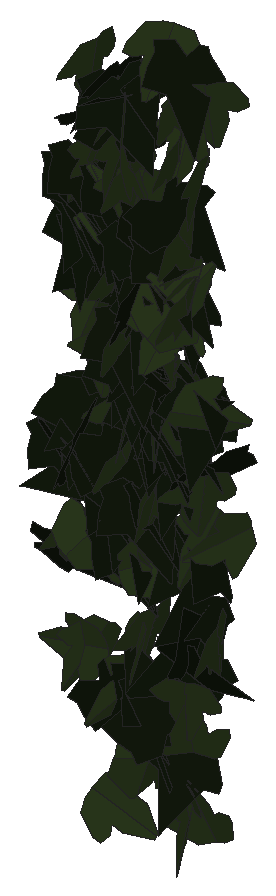
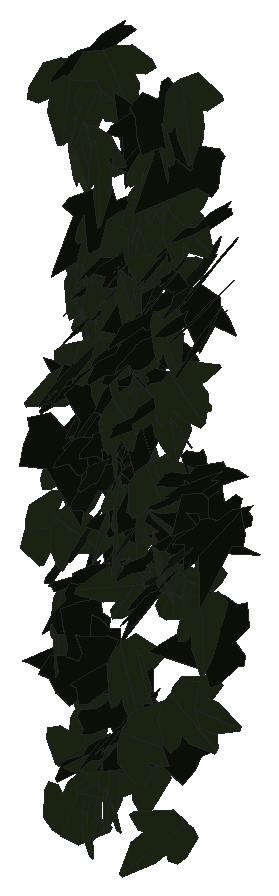
# SketchUp Ruby script. Lengths in inches.
U = 1.inch
M = Sketchup.active_model
def pt(a) = Geom::Point3d.new(a.map { |v| v * U })
def face(e, loops, mat)
  f = e.add_face(loops[0].map { |a| pt(a) })
  loops[1..].each { |l| e.add_face(l.map { |a| pt(a) }).erase! }
  f.material = f.back_material = mat if mat
  f
end
# faces: each face lists its corners as indices into pts; further lists are holes
def faces(e, pts, list, mat = nil) = list.each { |f| face(e, (f[0].is_a?(Array) ? f : [f]).map { |l| l.map { |i| pts[i] } }, mat) }
# xy, xz, yz: faces in a plane at the given z, y or x. An outline is a flat list of corners, or four numbers for a rectangle; further outlines are holes
def ring(l) = l.size == 4 ? [[l[0], l[1]], [l[2], l[1]], [l[2], l[3]], [l[0], l[3]]] : l.each_slice(2).to_a
def flat(e, list, mat, &to3) = list.each { |f| face(e, (f[0].is_a?(Array) ? f : [f]).map { |l| ring(l).map { |u, v| to3.(u, v) } }, mat) }
def xy(e, z, list, mat = nil) = flat(e, list, mat) { |x, y| [x, y, z] }
def xz(e, y, list, mat = nil) = flat(e, list, mat) { |x, z| [x, y, z] }
def yz(e, x, list, mat = nil) = flat(e, list, mat) { |y, z| [x, y, z] }
def lines(e, pts, list) = list.each { |a, b| e.add_line(pt(pts[a]), pt(pts[b])) }
# prism: a flat outline (further loops are holes) pulled along v
def prism(e, loops, v, mat = nil)
  f = face(e, loops, mat); d = Geom::Vector3d.new(v.map { |x| x * U })
  f.pushpull(f.normal.samedirection?(d) ? d.length : -d.length)
end
def box(e, o, s, mat = nil) = prism(e, [[o, [o[0] + s[0], o[1], o[2]], [o[0] + s[0], o[1] + s[1], o[2]], [o[0], o[1] + s[1], o[2]]]], [0, 0, s[2]], mat)
def at(x, y, z, deg = 0) = Geom::Transformation.translation(pt([x, y, z])) * Geom::Transformation.rotation(ORIGIN, Z_AXIS, deg.degrees)
def axes(o, x, y, z) = Geom::Transformation.new([*x, 0, *y, 0, *z, 0, *pt(o).to_a, 1])
def part(name) = M.definitions.add(name)
# library, detail: a bought-in or finely detailed component or shape, given as its bounding box
def library(name, o, s) = part(name).tap { |d| box(d.entities, o, s) }
def detail(e, o, s) = box(e.add_group.entities, o, s)
def put(e, d, t, mat = nil) = e.add_instance(d, t).tap { |i| i.material = mat if mat }
def group(e, t, mat = nil) = e.add_group.tap { |g| g.transformation = t; g.material = mat if mat }.entities
root = M.entities
M.materials.add("efeu1").color = [18, 25, 13]
M.materials.add("efeu2").color = [43, 57, 29]
c1 = part("ivyleaf_10")
p = [[0,0.5,-0.03],[-0.0625,2.02,-0.43],[-0.19,2.01,-0.46],[-0.54,1.05,-0.29],[-0.52,0.625,-0.18],[-0.83,0.76,-0.28],
  [-1.16,0.64,-0.33],[-1.15,0.33,-0.24],[-0.77,-0.39,0.02],[-0.3,-0.51,0.16],[0.04,-0.48,0.23],[-0.02,2.01,-0.4375],
  [-0.06,2.01,-0.43],[0.04,-0.49,0.23],[0.67,-0.49,0.14],[1.38,0.36,-0.2],[1.375,0.51,-0.24],[0.81,0.65,-0.19],
  [0.62,0.59,-0.15],[0.6,1.09,-0.28],[0.5,1.23,-0.31]]
faces(c1.entities,p,[[0,1,2,3,4,5,6,7,8,9,10],[11,12,0,13,14,15,16,17,18,19,20]],"efeu2")
c2 = part("ivyleaf_9")
p = [[1.54,2.16,1.25],[1.36,2.04,1.19],[-0.21,0.99,0.68],[-0.71,1.11,0.82],[-0.85,0.86,0.67],[-0.8,0.17,0.21],
  [-0.9,-0.01,0.1],[-0.67,-0.16,-0.02],[-0.08,-0.08,-0.05],[-0.03,-0.6,-0.4],[0.65,-0.88,-0.66],[0.83,-0.6,-0.49],
  [1.29,-0.42,-0.43],[1.8125,-0.07,-0.26],[1.21,0.44,0.15]]
faces(c2.entities,p,[[0,1,2,3,4,5,6,7,8,9,10,11,12,13,14]],"efeu1")
put(root,c1,axes([526.44,133.65,198.45],[0.31134,0.45715,-0.77984],[0.46763,0.62441,0.55273],[0.7736,-0.56142,-0.02027]))
put(root,c2,axes([527.04,134.69,195.85],[-0.12477,-0.77393,0.1001],[0.00797,-0.10263,-0.78355],[0.78033,-0.12269,0.02401]))
put(root,c1,axes([525.07,133.81,197.625],[-0.04112,-0.53898,-0.66297],[0.07443,0.65896,-0.54033],[0.85117,-0.08366,0.01522]))
put(root,c2,axes([526.71,134.58,188.76],[0.15218,0.40988,0.69617],[-0.23852,-0.65404,0.43722],[0.77186,-0.28292,-0.00215]))
put(root,c2,axes([525.39,133.55,198.23],[0.12896,0.35513,0.7991],[0.23978,0.76242,-0.37752],[-0.84094,0.27185,0.0149]))
put(root,c2,axes([525.3,134.86,194.29],[0.07511,-0.51258,0.6061],[0.11333,-0.59564,-0.51778],[0.78565,0.13493,0.01675]))
put(root,c1,axes([526.84,134.16,198.89],[0.0292,-0.79802,-0.29345],[0.04088,0.2946,-0.79708],[0.84928,0.01325,0.04846]))
put(root,c2,axes([526.11,134.29,186.49],[-0.63905,-0.58234,0.19141],[0.15334,0.11584,0.86442],[-0.5935,0.65697,0.01725]))
put(root,c2,axes([525.05,134.49,197.51],[-0.30421,-0.72268,-0.38636],[0.14579,0.35783,-0.78409],[0.8064,-0.33732,-0.004]))
put(root,c1,axes([526.21,134.41,198.08],[0.69804,0.27879,-0.29682],[-0.28882,-0.07628,-0.7509],[-0.28706,0.75468,0.03375]))
put(root,c2,axes([524.98,134.49,196.68],[-0.49657,-0.45951,-0.41466],[0.2841,0.30309,-0.67609],[0.54989,-0.57154,-0.02515]))
put(root,c2,axes([522.87,134.07,193.61],[0.6998,0.05372,-0.52183],[-0.5196,-0.04871,-0.70182],[-0.07217,0.87158,-0.00706]))
put(root,c2,axes([526.52,134.65,205.43],[0.02662,-0.84739,-0.0878],[-0.00156,0.0878,-0.84781],[0.85192,0.02664,0.00119]))
put(root,c2,axes([525.16,134.75,200.14],[0.2318,-0.75724,0.24907],[0.10266,-0.22887,-0.79136],[0.79051,0.25177,0.02974]))
put(root,c2,axes([525.83,134.49,199.98],[0.22908,-0.75036,-0.18724],[0.01233,0.1988,-0.7816],[0.77327,0.21913,0.06793]))
put(root,c2,axes([526.51,134.86,185.75],[-0.29078,-0.72484,0.15526],[-0.03642,-0.1526,-0.78067],[0.74039,-0.29218,0.02257]))
put(root,c1,axes([526.43,134.83,184.1],[0.2052,-0.48673,0.64315],[0.43004,-0.49542,-0.51213],[0.68236,0.45859,0.12936]))
put(root,c1,axes([523.77,134.41,204.93],[-0.06427,-0.83592,-0.05428],[0.00649,0.05394,-0.83838],[0.83766,-0.06455,0.00233]))
put(root,c2,axes([523.67,133.7,193.88],[-0.2778,0.34432,-0.75773],[-0.56075,0.51287,0.43864],[0.61504,0.62313,0.05767]))
put(root,c2,axes([523.3,134.75,194.66],[-0.39034,-0.6629,-0.13299],[0.11802,0.08441,-0.7671],[0.66573,-0.40365,0.05801]))
put(root,c1,axes([527.02,134.6,202.5625],[0.32017,-0.74024,0.1502],[0.09499,-0.12238,-0.80562],[0.74932,0.3318,0.03795]))
put(root,c1,axes([523.74,134.38,187.97],[0.13,0.01854,-0.7798],[-0.76876,0.13692,-0.1249],[0.13209,0.77862,0.04053]))
put(root,c2,axes([526.375,134.47,195.54],[0.56041,-0.56093,-0.02549],[-0.01663,0.01942,-0.7929],[0.56126,0.56065,0.00196]))
put(root,c1,axes([525.16,134.4,188.66],[0.50138,-0.62547,-0.22873],[-0.14537,0.17662,-0.80161],[0.64992,0.52202,-0.00284]))
put(root,c1,axes([524.48,134.71,202.5],[0.15512,-0.7754,0.28206],[0.09573,-0.26815,-0.78981],[0.81954,0.17809,0.03887]))
put(root,c1,axes([527.09,133.92,196.01],[-0.23757,-0.29741,-0.81773],[0.54563,0.60938,-0.38016],[0.67781,-0.59479,0.01941]))
put(root,c1,axes([526.73,134.38,187.72],[-0.7022,-0.23546,0.06145],[-0.0567,-0.0242,-0.74061],[0.23665,-0.70447,0.00491]))
put(root,c1,axes([523.58,134.82,188.09],[-0.15948,-0.64811,0.46925],[-0.07214,-0.46488,-0.66659],[0.79689,-0.17179,0.03357]))
put(root,c1,axes([523.62,133.95,191.07],[0.3816,0.27253,-0.68362],[0.46599,0.50654,0.46206],[0.56961,-0.59697,0.07998]))
put(root,c2,axes([524.44,134.53,204.55],[-0.33256,0.6112,-0.43787],[0.12378,-0.42775,-0.69109],[-0.7416,-0.34548,0.081]))
put(root,c1,axes([524.07,134.5,191.02],[-0.01847,-0.04676,0.81979],[0.82026,0.03653,0.02056],[-0.03764,0.81918,0.04588]))
put(root,c1,axes([524.74,134.63,195.1],[0.48288,-0.61856,0.09808],[0.05435,-0.08199,-0.78469],[0.62392,0.48588,-0.00755]))
put(root,c1,axes([527.17,134.5,193.68],[-0.42602,-0.67903,0.04435],[-0.02532,-0.03647,-0.8016],[0.68,-0.42676,-0.00206]))
put(root,c2,axes([523.24,134.63,201.55],[0.15948,-0.78413,-0.19331],[0.01342,0.19959,-0.79853],[0.8075,0.15155,0.05145]))
put(root,c1,axes([524.23,134.67,198.63],[0.18506,-0.79542,0.11417],[0.03765,-0.10845,-0.81658],[0.80269,0.18848,0.01198]))
put(root,c2,axes([526.82,135.16,190.1],[0.19036,-0.31801,-0.71542],[0.32402,-0.63825,0.36992],[-0.71272,-0.3751,-0.02291]))
put(root,c1,axes([526.44,134.45,199.09],[-0.27492,-0.77628,-0.1375],[0.05103,0.12779,-0.82351],[0.78671,-0.27956,0.00536]))
put(root,c2,axes([524.61,134.27,202.73],[-0.45695,-0.09896,0.70036],[0.70193,0.03932,0.46352],[-0.08718,0.83532,0.06115]))
put(root,c2,axes([525.76,134.51,195.24],[0.1186,-0.16988,0.8106],[0.77965,-0.25337,-0.16717],[0.27942,0.77907,0.12239]))
put(root,c2,axes([525.26,134.64,187.14],[0.30181,-0.71253,-0.15559],[-0.03025,0.15602,-0.77314],[0.72869,0.30159,0.03235]))
put(root,c1,axes([524.39,134.1,184.01],[0.27208,0.45753,0.6261],[0.30847,0.5449,-0.53225],[-0.71146,0.41123,0.00867]))
put(root,c1,axes([523.51,134.97,201.84],[0.05713,-0.63947,0.49199],[0.05244,-0.48924,-0.64198],[0.80512,0.07724,0.0069]))
put(root,c2,axes([524.5,134.5,204.14],[-0.13046,-0.62877,-0.56176],[0.07364,0.55778,-0.64141],[0.83994,-0.14656,-0.03102]))
put(root,c2,axes([525.72,134.99,194.38],[0.21799,-0.64149,0.45015],[0.21823,-0.39907,-0.67437],[0.75267,0.30149,0.06516]))
put(root,c2,axes([525.13,134.57,192.73],[-0.20018,-0.57923,-0.54341],[0.22082,0.49772,-0.61187],[0.76292,-0.29604,0.03452]))
put(root,c2,axes([523.91,135.04,199.85],[0.1509,-0.68165,0.39536],[0.11026,-0.38032,-0.6978],[0.78025,0.18558,0.02215]))
put(root,c2,axes([524.2,134.27,194.06],[-0.00202,-0.34703,-0.79748],[0.20834,0.77407,-0.33738],[0.84439,-0.19182,0.08133]))
put(root,c1,axes([525.22,134.06,185.55],[-0.15506,-0.17635,-0.85934],[0.63317,0.5815,-0.23358],[0.60717,-0.65144,0.02413]))
put(root,c2,axes([526.9,135.07,196.23],[0.08953,-0.6586,0.46324],[0.21512,-0.42959,-0.65233],[0.77594,0.19509,0.12741]))
put(root,c2,axes([525.14,134.33,196.5],[-0.46457,0.53391,0.36751],[-0.28183,0.24078,-0.70607],[-0.58368,-0.54121,0.04842]))
put(root,c1,axes([525.34,135.0625,194.79],[0.09278,-0.30387,0.75573],[0.55167,-0.53617,-0.28332],[0.59928,0.54062,0.1438]))
put(root,c2,axes([524.05,134.9,192.87],[-0.63778,-0.06359,0.51912],[-0.5109,-0.09932,-0.63985],[0.11184,-0.81633,0.03741]))
put(root,c2,axes([526.8,135.22,191.27],[-0.06868,-0.54907,0.63036],[0.13004,-0.63181,-0.53616],[0.82579,0.05383,0.13685]))
put(root,c2,axes([523.04,135.04,200.21],[0.21505,-0.71302,0.35637],[0.1455,-0.3278,-0.74365],[0.78372,0.2565,0.04027]))
put(root,c1,axes([526.86,135.15,192.16],[-0.08458,-0.55649,0.62678],[0.18393,-0.62693,-0.53181],[0.81774,0.08345,0.18444]))
put(root,c1,axes([526.36,134.49,196.79],[-0.76986,0.10412,0.33772],[-0.33872,0.01357,-0.77632],[-0.10083,-0.84057,0.0293]))
put(root,c2,axes([526.78,134.99,188.44],[-0.00772,-0.02878,-0.80378],[-0.33633,-0.73005,0.02937],[-0.7306,0.33638,-0.00502]))
put(root,c1,axes([526.625,134.81,199],[-0.00456,-0.80127,0.13001],[-0.01809,-0.12988,-0.8011],[0.81155,-0.0074,-0.01712]))
put(root,c2,axes([525.87,134.67,199.47],[0.33139,-0.69883,-0.2613],[0.03236,0.29911,-0.75891],[0.74538,0.29771,0.14911]))
put(root,c1,axes([526.59,134.86,185.74],[-0.4981,-0.6166,-0.17507],[-0.10956,-0.13655,0.79266],[-0.63154,0.51001,0.00057]))
put(root,c2,axes([522.23,134.52,190.29],[0.66453,-0.16089,0.42007],[0.41368,-0.07577,-0.68343],[0.17669,0.78251,0.02019]))
put(root,c1,axes([525.2,134.93,199.42],[0.2443,-0.70608,0.29635],[0.18362,-0.24797,-0.74219],[0.74341,0.29328,0.08593]))
put(root,c2,axes([524.3,134.59,191.37],[0.34255,-0.65099,-0.38619],[-0.14454,0.35984,-0.73478],[0.743,0.37013,0.03511]))
put(root,c1,axes([524.59,135.24,187.03],[-0.07132,-0.4363,0.75754],[-0.11677,-0.74849,-0.44209],[0.86637,-0.1368,0.00278]))
put(root,c2,axes([523.2,134.84,199.88],[-0.61832,-0.20887,-0.52588],[0.48542,0.20449,-0.65196],[0.29077,-0.78553,-0.02989]))
put(root,c2,axes([523.73,134.03,203.33],[0.5432,0.54528,0.27712],[0.04991,0.32988,-0.74691],[-0.60962,0.51287,0.18578]))
put(root,c1,axes([524.14,134.72,196.48],[-0.64908,-0.41453,0.17804],[-0.12739,-0.13085,-0.76908],[0.43279,-0.66021,0.04064]))
put(root,c2,axes([526.19,134.93,194.29],[-0.66044,-0.28531,-0.38832],[0.36993,0.12198,-0.71878],[0.30879,-0.75637,0.03056]))
put(root,c2,axes([526.2,134.59,188.3],[0.5605,-0.13073,0.50882],[0.48668,-0.15095,-0.5749],[0.19782,0.74181,-0.02732]))
put(root,c2,axes([524.72,135.17,191.28],[0.11723,-0.67059,0.38038],[0.04206,-0.37861,-0.68045],[0.76981,0.12281,-0.02075]))
put(root,c1,axes([524.23,134.8,192.39],[0.30376,-0.70834,0.0458],[0.02472,-0.03923,-0.77069],[0.70939,0.30468,0.00725]))
put(root,c2,axes([525.01,134.38,196.31],[0.50677,0.45524,-0.40751],[-0.38605,-0.17179,-0.672],[-0.47358,0.62719,0.11172]))
put(root,c2,axes([523.56,135.28,192.25],[-0.15692,-0.61523,0.48098],[0.12926,-0.50429,-0.60287],[0.77016,-0.04072,0.19919]))
put(root,c2,axes([525.33,134.99,195.2],[-0.27321,-0.74959,-0.16478],[0.04275,0.15977,-0.79769],[0.76629,-0.27616,-0.01424]))
put(root,c2,axes([522.51,134.74,193.6],[0.08383,-0.67692,-0.36171],[0.05206,0.36804,-0.6767],[0.76573,0.04909,0.0856]))
put(root,c2,axes([524.97,134.57,200.1],[0.12897,-0.58757,-0.57627],[0.01112,0.5845,-0.59347],[0.82292,0.08419,0.09833]))
put(root,c1,axes([527.08,134.84,183.72],[-0.7173,-0.11572,-0.25862],[-0.25255,-0.05795,0.7264],[-0.12843,0.76029,0.016]))
put(root,c2,axes([524.08,134.36,187.08],[-0.00997,-0.00816,-0.79816],[0.36214,0.7113,-0.01179],[0.71133,-0.36224,-0.00518]))
put(root,c2,axes([526.18,134.95,194.74],[-0.07352,-0.74961,-0.20474],[-0.00945,0.2065,-0.75267],[0.77701,-0.06842,-0.02853]))
put(root,c2,axes([525.37,135.11,186.9],[0.12094,-0.86457,0.05842],[0.01008,-0.05758,-0.87298],[0.86648,0.12135,0.002]))
put(root,c1,axes([524.89,134.41,202.24],[-0.27544,0.69997,0.30219],[-0.14771,0.26623,-0.7513],[-0.74797,-0.31034,0.03709]))
put(root,c1,axes([525.61,134.47,192.89],[0.17255,-0.71204,-0.44932],[0.00788,0.46,-0.72594],[0.84191,0.14163,0.09888]))
put(root,c1,axes([526.62,134.84,199.35],[0.53244,-0.61331,-0.0153],[-0.01234,0.00955,-0.81218],[0.61337,0.53258,-0.00306]))
put(root,c2,axes([524.33,135.2,192.25],[-0.15891,-0.73599,0.14313],[0.01693,-0.14979,-0.75147],[0.74959,-0.15265,0.04732]))
put(root,c1,axes([524.25,134.74,200.02],[0.36318,0.69126,0.2309],[-0.16386,-0.17393,0.77843],[0.71014,-0.39365,0.06152]))
put(root,c1,axes([524.625,134.53,193.6],[-0.16599,-0.69127,-0.35294],[0.07547,0.34484,-0.71089],[0.77248,-0.18223,-0.00639]))
put(root,c2,axes([523.79,134.96,200.9],[0.30086,-0.772,-0.06699],[-0.01959,0.06427,-0.82854],[0.77465,0.30146,0.00507]))
put(root,c2,axes([527.42,134.55,194.34],[0.04036,0.75873,-0.26869],[-0.04809,-0.26628,-0.75913],[-0.80346,0.05405,0.03194]))
put(root,c2,axes([522.51,135,200.77],[0.30613,-0.76598,-0.00762],[-0.00116,0.00774,-0.82489],[0.76602,0.30613,0.0018]))
put(root,c2,axes([522.82,135.4,198.45],[-0.11527,-0.45927,0.64404],[-0.07346,-0.64181,-0.47083],[0.7876,-0.12708,0.05035]))
put(root,c1,axes([524.41,134.6,203.65],[0.57685,-0.50635,-0.3483],[-0.14174,0.3552,-0.75113],[0.598,0.57262,0.15794]))
put(root,c1,axes([525.82,134.58,185.68],[0.08938,-0.76116,-0.33495],[0.04447,0.34077,-0.76252],[0.83041,0.06368,0.07688]))
put(root,c1,axes([526.48,134.47,200.47],[-0.00699,-0.65575,-0.47411],[0.07301,0.47168,-0.65347],[0.80588,-0.04842,0.05509]))
put(root,c1,axes([527.42,134.65,189.46],[0.17474,-0.73806,-0.29627],[0.02007,0.30734,-0.75378],[0.79505,0.15446,0.08414]))
put(root,c2,axes([523.38,135.42,194.3125],[-0.46747,-0.46715,0.42333],[-0.11137,-0.45753,-0.62787],[0.62051,-0.43405,0.20623]))
put(root,c2,axes([525.75,135.32,193.72],[0.03386,-0.50671,0.63045],[0.29979,-0.5782,-0.48081],[0.75123,0.25358,0.16346]))
put(root,c2,axes([525.05,134.9,192.48],[0.44622,-0.62635,-0.09543],[-0.04331,0.08629,-0.7689],[0.63209,0.44808,0.01468]))
put(root,c2,axes([525.93,134.49,201.22],[-0.0308,-0.3485,-0.76476],[0.0344,0.76411,-0.34959],[0.83972,-0.04408,-0.01373]))
put(root,c1,axes([526.41,134.6,184.99],[-0.59935,0.31923,0.27874],[-0.24105,0.14031,-0.67899],[-0.34857,-0.64593,-0.00973]))
put(root,c1,axes([524.78,134.62,201.68],[-0.07943,-0.74912,-0.37046],[0.0976,0.36127,-0.75146],[0.83,-0.11417,0.05291]))
put(root,c2,axes([525.13,135.33,197.67],[-0.17567,-0.77637,0.16821],[-0.05905,-0.15904,-0.7957],[0.79219,-0.18402,-0.02201]))
put(root,c1,axes([522.89,134.82,191.02],[-0.17029,-0.73889,-0.09967],[0.00759,0.10052,-0.75811],[0.74554,-0.16979,-0.01505]))
put(root,c1,axes([525.33,135.18,184.95],[-0.022,0.0285,0.83238],[0.76008,-0.33976,0.03172],[0.34053,0.7602,-0.01703]))
put(root,c1,axes([525.67,134.46,193.11],[0.02992,-0.61439,-0.60164],[0.13107,0.59823,-0.60439],[0.84987,-0.07063,0.11439]))
put(root,c1,axes([525.23,134.29,190.76],[-0.0224,-0.11945,0.83068],[0.2347,0.79693,0.12092],[-0.80574,0.23545,0.01213]))
put(root,c1,axes([525.57,134.99,199.38],[-0.30972,-0.76156,0.08257],[0.01179,-0.09379,-0.82084],[0.76593,-0.30651,0.04602]))
put(root,c1,axes([525.08,135.05,188.92],[0.04416,-0.92118,0.08716],[0.01501,-0.08654,-0.92217],[0.92517,0.04537,0.0108]))
put(root,c1,axes([524.8125,135.02,201.25],[-0.5889,-0.54754,0.16804],[-0.05024,-0.19071,-0.79746],[0.57053,-0.58196,0.10323]))
put(root,c1,axes([524.43,134.64,202.9],[-0.23781,-0.69392,-0.40727],[0.13592,0.38394,-0.73353],[0.79305,-0.27389,0.0036]))
put(root,c1,axes([525.625,135,205.5625],[0.68844,0.41131,-0.22014],[-0.20171,-0.0914,-0.80159],[-0.42066,0.71697,0.0241]))
put(root,c1,axes([527.02,134.85,204.54],[-0.65434,-0.52079,-0.06307],[0.04535,0.04429,-0.83626],[0.52263,-0.65587,-0.0064]))
put(root,c1,axes([526.32,134.55,204.28],[-0.0472,-0.62052,-0.55209],[0.14995,0.53752,-0.61697],[0.81692,-0.13452,0.08135]))
put(root,c1,axes([527.55,135.42,192.01],[0.02986,0.15929,-0.76146],[-0.43898,-0.62565,-0.1481],[-0.64225,0.43505,0.06582]))
put(root,c2,axes([524.08,135.2,198.42],[0.10408,-0.80532,-0.11078],[0.00204,0.11194,-0.81186],[0.81291,0.10283,0.01622]))
put(root,c2,axes([524.45,135.47,196.22],[-0.22394,-0.72771,0.22445],[-0.0338,-0.22422,-0.76071],[0.76079,-0.22416,0.03227]))
put(root,c2,axes([524.35,135.39,199],[-0.0547,-0.79723,0.10403],[-0.02244,-0.10271,-0.79896],[0.80367,-0.05712,-0.01523]))
put(root,c1,axes([526.17,135.02,203.22],[0.80109,-0.17079,-0.0484],[-0.03764,0.05522,-0.8178],[0.17348,0.80065,0.04608]))
put(root,c1,axes([525.01,135.33,196.07],[-0.18359,-0.65614,0.39725],[-0.0415,-0.39937,-0.67883],[0.7659,-0.17892,0.05844]))
put(root,c2,axes([524.14,135.1,191.25],[0.27206,-0.69458,-0.17136],[-0.02874,0.17257,-0.74513],[0.71483,0.27129,0.03526]))
put(root,c2,axes([522.64,135.59,199.53],[-0.12065,-0.66474,0.43452],[0.04258,-0.44429,-0.66786],[0.79301,-0.07728,0.10197]))
put(root,c2,axes([525.42,135.37,199.65],[0.23912,-0.76209,0.16662],[0.02922,-0.1654,-0.79845],[0.77955,0.23997,-0.02118]))
put(root,c1,axes([526.02,134.86,202.67],[0.14867,-0.77014,-0.30489],[-0.01789,0.30671,-0.78345],[0.8281,0.14489,0.03782]))
put(root,c2,axes([525.97,135.43,198.41],[0.10309,-0.77423,0.18754],[0.06045,-0.18095,-0.78028],[0.79432,0.11425,0.03504]))
put(root,c1,axes([524.1,135.25,194.46],[-0.27784,-0.67667,0.26113],[-0.04329,-0.26367,-0.72929],[0.72401,-0.27544,0.05661]))
put(root,c1,axes([523.18,135.43,197.51],[-0.26492,-0.62399,0.42829],[0.08749,-0.47597,-0.63936],[0.75176,-0.1645,0.22534]))
put(root,c2,axes([526.22,135.61,191.17],[-0.47203,-0.54266,0.27252],[-0.02645,-0.32646,-0.6959],[0.60667,-0.43646,0.18169]))
